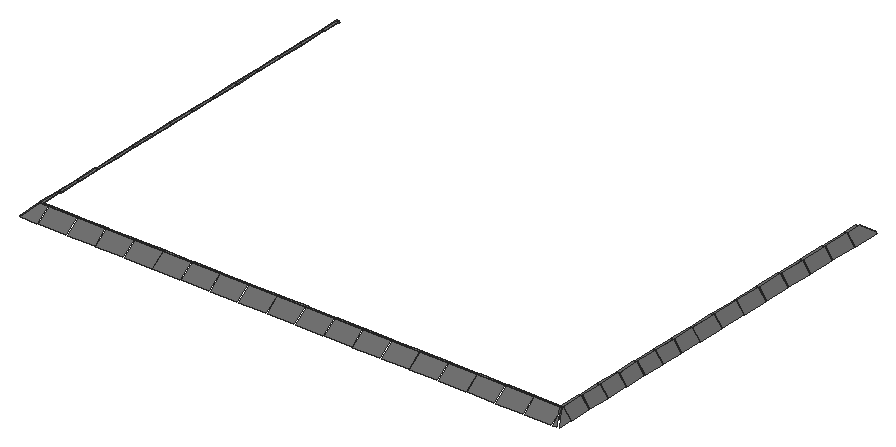
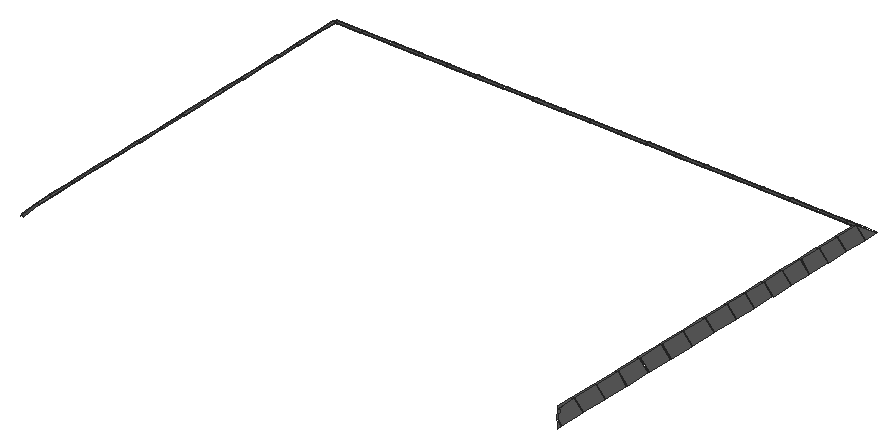
# SketchUp Ruby script. Lengths in inches.
U = 1.inch
M = Sketchup.active_model
def pt(a) = Geom::Point3d.new(a.map { |v| v * U })
def face(e, loops, mat)
  f = e.add_face(loops[0].map { |a| pt(a) })
  loops[1..].each { |l| e.add_face(l.map { |a| pt(a) }).erase! }
  f.material = f.back_material = mat if mat
  f
end
# faces: each face lists its corners as indices into pts; further lists are holes
def faces(e, pts, list, mat = nil) = list.each { |f| face(e, (f[0].is_a?(Array) ? f : [f]).map { |l| l.map { |i| pts[i] } }, mat) }
# xy, xz, yz: faces in a plane at the given z, y or x. An outline is a flat list of corners, or four numbers for a rectangle; further outlines are holes
def ring(l) = l.size == 4 ? [[l[0], l[1]], [l[2], l[1]], [l[2], l[3]], [l[0], l[3]]] : l.each_slice(2).to_a
def flat(e, list, mat, &to3) = list.each { |f| face(e, (f[0].is_a?(Array) ? f : [f]).map { |l| ring(l).map { |u, v| to3.(u, v) } }, mat) }
def xy(e, z, list, mat = nil) = flat(e, list, mat) { |x, y| [x, y, z] }
def xz(e, y, list, mat = nil) = flat(e, list, mat) { |x, z| [x, y, z] }
def yz(e, x, list, mat = nil) = flat(e, list, mat) { |y, z| [x, y, z] }
def lines(e, pts, list) = list.each { |a, b| e.add_line(pt(pts[a]), pt(pts[b])) }
# prism: a flat outline (further loops are holes) pulled along v
def prism(e, loops, v, mat = nil)
  f = face(e, loops, mat); d = Geom::Vector3d.new(v.map { |x| x * U })
  f.pushpull(f.normal.samedirection?(d) ? d.length : -d.length)
end
def box(e, o, s, mat = nil) = prism(e, [[o, [o[0] + s[0], o[1], o[2]], [o[0] + s[0], o[1] + s[1], o[2]], [o[0], o[1] + s[1], o[2]]]], [0, 0, s[2]], mat)
def at(x, y, z, deg = 0) = Geom::Transformation.translation(pt([x, y, z])) * Geom::Transformation.rotation(ORIGIN, Z_AXIS, deg.degrees)
def axes(o, x, y, z) = Geom::Transformation.new([*x, 0, *y, 0, *z, 0, *pt(o).to_a, 1])
def part(name) = M.definitions.add(name)
# library, detail: a bought-in or finely detailed component or shape, given as its bounding box
def library(name, o, s) = part(name).tap { |d| box(d.entities, o, s) }
def detail(e, o, s) = box(e.add_group.entities, o, s)
def put(e, d, t, mat = nil) = e.add_instance(d, t).tap { |i| i.material = mat if mat }
def group(e, t, mat = nil) = e.add_group.tap { |g| g.transformation = t; g.material = mat if mat }.entities
root = M.entities
M.materials.add("[Color M05]").color = [114, 114, 114]
p = [[790.34,286.64,408.32],[790.34,298,408.32],[783.88,298,416.64],[785.7,294.8,414.29],[787.2,292.16,412.36],[790.34,299.21,408.32],
  [790.34,317.375,408.32],[783.88,317.375,416.64],[783.88,299.21,416.64],[790.34,318.58,408.32],[790.34,336.74,408.32],[783.88,336.74,416.64],
  [783.88,318.58,416.64],[790.34,337.95,408.32],[790.34,356.11,408.32],[783.88,356.11,416.64],[783.88,337.95,416.64],[790.34,357.32,408.32],
  [790.34,375.48,408.32],[783.88,375.48,416.64],[783.88,357.32,416.64],[790.34,376.69,408.32],[790.34,394.85,408.32],[783.88,394.85,416.64],
  [783.88,376.69,416.64],[790.34,396.0625,408.32],[790.34,414.22,408.32],[783.88,414.22,416.64],[783.88,396.0625,416.64],[790.34,415.43,408.32],
  [790.34,433.59,408.32],[783.88,433.59,416.64],[783.88,415.43,416.64],[790.34,434.8,408.32],[790.34,456.8,408.32],[783.88,456.8,416.64],
  [783.88,434.8,416.64],[790.34,458.01,408.32],[790.34,480.02,408.32],[783.88,480.02,416.64],[783.88,458.01,416.64],[790.34,481.23,408.32],
  [790.34,503.23,408.32],[783.88,503.23,416.64],[783.88,481.23,416.64],[790.34,504.44,408.32],[790.34,526.45,408.32],[783.88,526.45,416.64],
  [783.88,504.44,416.64],[790.34,527.66,408.32],[790.34,549.66,408.32],[783.88,549.66,416.64],[783.88,527.66,416.64],[790.34,550.87,408.32],
  [790.34,572.875,408.32],[783.88,572.875,416.64],[783.88,550.87,416.64],[790.34,574.08,408.32],[790.34,596.09,408.32],[783.88,596.09,416.64],
  [783.88,574.08,416.64],[790.34,597.3,408.32],[790.34,619.3,408.32],[788.98,619.3,410.08],[783.88,610.34,416.64],[783.88,597.3,416.64],
  [336.88,286.64,408.43],[344.33,298,416.75],[336.88,298,408.43],[336.88,317.375,408.43],[336.88,299.21,408.43],[344.33,299.21,416.75],
  [344.33,317.375,416.75],[336.88,336.74,408.43],[336.88,318.58,408.43],[344.33,318.58,416.75],[344.33,336.74,416.75],[336.88,356.11,408.43],
  [336.88,337.95,408.43],[344.33,337.95,416.75],[344.33,356.11,416.75],[336.88,375.48,408.43],[336.88,357.32,408.43],[344.33,357.32,416.75],
  [344.33,375.48,416.75],[336.88,394.85,408.43],[336.88,376.69,408.43],[344.33,376.69,416.75],[344.33,394.85,416.75],[336.88,414.22,408.43],
  [336.88,396.0625,408.43],[344.33,396.0625,416.75],[344.33,414.22,416.75],[336.88,433.3,408.43],[336.88,415.43,408.43],[344.33,415.43,416.75],
  [344.33,433.3,416.75],[344.33,434.8,416.75],[344.33,456.21,416.75],[336.88,456.21,408.43],[336.88,434.8,408.43],[336.88,479.13,408.43],
  [336.88,457.71,408.43],[344.33,457.71,416.75],[344.33,479.13,416.75],[336.88,502.04,408.43],[336.88,480.63,408.43],[344.33,480.63,416.75],
  [344.33,502.04,416.75],[336.88,524.95,408.43],[336.88,503.54,408.43],[344.33,503.54,416.75],[344.33,524.95,416.75],[336.88,547.87,408.43],
  [336.88,526.45,408.43],[344.33,526.45,416.75],[344.33,547.87,416.75],[336.88,570.78,408.43],[336.88,549.37,408.43],[344.33,549.37,416.75],
  [344.33,570.78,416.75],[336.88,593.69,408.43],[336.88,572.28,408.43],[344.33,572.28,416.75],[344.33,593.69,416.75],[336.88,616.61,408.43],
  [336.88,595.19,408.43],[344.33,595.19,416.75],[344.33,610.34,416.75],[340.22,616.61,412.16],[336.88,621.71,408.43],[336.88,618.11,408.43],
  [339.24,618.11,411.06],[338.37,285.45,408.71],[352.12,285.45,408.71],[352.12,296.82,417.03],[345.82,296.82,417.03],[353.62,285.45,408.71],
  [376.12,285.45,408.71],[376.12,296.82,417.03],[353.62,296.82,417.03],[377.62,285.45,408.71],[400.12,285.45,408.71],[400.12,296.82,417.03],
  [377.62,296.82,417.03],[401.62,285.45,408.71],[424.12,285.45,408.71],[424.12,296.82,417.03],[401.62,296.82,417.03],[425.62,285.45,408.71],
  [448.12,285.45,408.71],[448.12,296.82,417.03],[425.62,296.82,417.03],[449.62,285.45,408.71],[472.12,285.45,408.71],[472.12,296.82,417.03],
  [449.62,296.82,417.03],[473.62,285.45,408.71],[496.12,285.45,408.71],[496.12,296.82,417.03],[473.62,296.82,417.03],[497.62,285.45,408.71],
  [520.12,285.45,408.71],[520.12,296.82,417.03],[497.62,296.82,417.03],[521.62,285.45,408.71],[544.12,285.45,408.71],[544.12,296.82,417.03],
  [521.62,296.82,417.03],[545.62,285.45,408.71],[568.12,285.45,408.71],[568.12,296.82,417.03],[545.62,296.82,417.03],[569.62,285.45,408.71],
  [592.12,285.45,408.71],[592.12,296.82,417.03],[569.62,296.82,417.03],[593.62,285.45,408.71],[616.15,285.45,408.71],[616.15,296.82,417.03],
  [593.62,296.82,417.03],[617.62,285.45,408.71],[640.12,285.45,408.71],[640.12,296.82,417.03],[617.62,296.82,417.03],[641.62,285.45,408.71],
  [664.12,285.45,408.71],[664.12,296.82,417.03],[641.62,296.82,417.03],[665.62,285.45,408.71],[688.12,285.45,408.71],[688.12,296.82,417.03],
  [665.62,296.82,417.03],[689.62,285.45,408.71],[712.12,285.45,408.71],[712.12,296.82,417.03],[689.62,296.82,417.03],[713.62,285.45,408.71],
  [736.12,285.45,408.71],[736.12,296.82,417.03],[713.62,296.82,417.03],[737.62,285.45,408.71],[760.12,285.45,408.71],[760.12,296.82,417.03],
  [737.62,296.82,417.03],[761.62,285.45,408.71],[784.12,285.45,408.71],[784.12,293.62,414.68],[782.3,296.82,417.03],[761.62,296.82,417.03],
  [788.76,285.45,408.71],[785.62,290.98,412.75],[785.62,285.45,408.71],[787.4,619.3,408.85],[782.3,610.34,415.41],[345.82,610.34,415.41],
  [341.71,616.61,410.82],[784.12,294.8,413.07],[785.62,292.16,411.14],[782.3,298,415.41],[352.12,298,415.41],[345.82,298,415.41],
  [376.12,298,415.41],[353.62,298,415.41],[400.12,298,415.41],[377.62,298,415.41],[424.12,298,415.41],[401.62,298,415.41],
  [448.12,298,415.41],[425.62,298,415.41],[472.12,298,415.41],[449.62,298,415.41],[496.12,298,415.41],[473.62,298,415.41],
  [520.12,298,415.41],[497.62,298,415.41],[544.12,298,415.41],[521.62,298,415.41],[568.12,298,415.41],[545.62,298,415.41],
  [592.12,298,415.41],[569.62,298,415.41],[616.15,298,415.41],[593.62,298,415.41],[640.12,298,415.41],[617.62,298,415.41],
  [664.12,298,415.41],[641.62,298,415.41],[688.12,298,415.41],[665.62,298,415.41],[712.12,298,415.41],[689.62,298,415.41],
  [736.12,298,415.41],[713.62,298,415.41],[760.12,298,415.41],[737.62,298,415.41],[761.62,298,415.41],[352.12,299.21,416.3],
  [346.61,299.21,416.3],[345.82,299.21,415.41],[353.62,299.21,416.3],[376.12,299.21,416.3],[377.62,299.21,416.3],[400.12,299.21,416.3],
  [401.62,299.21,416.3],[424.12,299.21,416.3],[425.62,299.21,416.3],[448.12,299.21,416.3],[449.62,299.21,416.3],[472.12,299.21,416.3],
  [473.62,299.21,416.3],[496.12,299.21,416.3],[497.62,299.21,416.3],[520.12,299.21,416.3],[521.62,299.21,416.3],[544.12,299.21,416.3],
  [545.62,299.21,416.3],[568.12,299.21,416.3],[569.62,299.21,416.3],[592.12,299.21,416.3],[593.62,299.21,416.3],[616.15,299.21,416.3],
  [617.62,299.21,416.3],[640.12,299.21,416.3],[641.62,299.21,416.3],[664.12,299.21,416.3],[665.62,299.21,416.3],[688.12,299.21,416.3],
  [689.62,299.21,416.3],[712.12,299.21,416.3],[713.62,299.21,416.3],[736.12,299.21,416.3],[737.62,299.21,416.3],[760.12,299.21,416.3],
  [761.62,299.21,416.3],[781.61,299.21,416.3],[782.3,299.21,415.41],[345.82,317.375,415.41],[346.61,317.375,416.3],[782.3,317.375,415.41],
  [781.61,317.375,416.3],[345.82,318.58,415.41],[346.61,318.58,416.3],[782.3,318.58,415.41],[781.61,318.58,416.3],[345.82,336.74,415.41],
  [346.61,336.74,416.3],[782.3,336.74,415.41],[781.61,336.74,416.3],[345.82,337.95,415.41],[346.61,337.95,416.3],[782.3,337.95,415.41],
  [781.61,337.95,416.3],[345.82,356.11,415.41],[346.61,356.11,416.3],[782.3,356.11,415.41],[781.61,356.11,416.3],[345.82,357.32,415.41],
  [346.61,357.32,416.3],[782.3,357.32,415.41],[781.61,357.32,416.3],[345.82,375.48,415.41],[346.61,375.48,416.3],[782.3,375.48,415.41],
  [781.61,375.48,416.3],[346.61,376.69,416.3],[345.82,376.69,415.41],[782.3,376.69,415.41],[781.61,376.69,416.3],[345.82,394.85,415.41],
  [346.61,394.85,416.3],[782.3,394.85,415.41],[781.61,394.85,416.3],[345.82,396.0625,415.41],[346.61,396.0625,416.3],[782.3,396.0625,415.41],
  [781.61,396.0625,416.3],[345.82,414.22,415.41],[346.61,414.22,416.3],[782.3,414.22,415.41],[781.61,414.22,416.3],[345.82,415.43,415.41],
  [346.61,415.43,416.3],[782.3,415.43,415.41],[781.61,415.43,416.3],[345.82,433.3,415.41],[346.61,433.3,416.3],[782.3,433.59,415.41],
  [781.61,433.59,416.3],[345.82,434.8,415.41],[346.61,434.8,416.3],[782.3,434.8,415.41],[781.61,434.8,416.3],[345.82,456.21,415.41],
  [346.61,456.21,416.3],[782.3,456.8,415.41],[781.61,456.8,416.3],[345.82,457.71,415.41],[346.61,457.71,416.3],[782.3,458.01,415.41],
  [781.61,458.01,416.3],[345.82,479.13,415.41],[346.61,479.13,416.3],[782.3,480.02,415.41],[781.61,480.02,416.3],[345.82,480.63,415.41],
  [346.61,480.63,416.3],[782.3,481.23,415.41],[781.61,481.23,416.3],[345.82,502.04,415.41],[346.61,502.04,416.3],[782.3,503.23,415.41],
  [781.61,503.23,416.3],[345.82,503.54,415.41],[346.61,503.54,416.3],[782.3,504.44,415.41],[781.61,504.44,416.3],[345.82,524.95,415.41],
  [346.61,524.95,416.3],[782.3,526.45,415.41],[781.61,526.45,416.3],[345.82,526.45,415.41],[346.61,526.45,416.3],[782.3,527.66,415.41],
  [781.61,527.66,416.3],[345.82,547.87,415.41],[346.61,547.87,416.3],[782.3,549.66,415.41],[781.61,549.66,416.3],[345.82,549.37,415.41],
  [346.61,549.37,416.3],[345.82,570.78,415.41],[346.61,570.78,416.3],[782.3,550.87,415.41],[781.61,550.87,416.3],[782.3,572.875,415.41],
  [781.61,572.875,416.3],[345.82,572.28,415.41],[346.61,572.28,416.3],[345.82,593.69,415.41],[346.61,593.69,416.3],[782.3,574.08,415.41],
  [781.61,574.08,416.3],[782.3,596.09,415.41],[781.61,596.09,416.3],[345.82,595.19,415.41],[346.61,595.19,416.3],[346.61,609.125,416.3],
  [782.3,597.3,415.41],[781.61,597.3,416.3],[781.61,609.125,416.3]]
faces(root,p,[[0,1,2,3,4],[5,6,7,8],[9,10,11,12],[13,14,15,16],[17,18,19,20],[21,22,23,24],[25,26,27,28],[29,30,31,32],
  [33,34,35,36],[37,38,39,40],[41,42,43,44],[45,46,47,48],[49,50,51,52],[53,54,55,56],[57,58,59,60],[61,62,63,64,65],
  [66,67,68],[69,70,71,72],[73,74,75,76],[77,78,79,80],[81,82,83,84],[85,86,87,88],[89,90,91,92],[93,94,95,96],
  [97,98,99,100],[101,102,103,104],[105,106,107,108],[109,110,111,112],[113,114,115,116],[117,118,119,120],[121,122,123,124],[125,126,127,128,129],
  [130,131,132],[133,134,135,136],[137,138,139,140],[141,142,143,144],[145,146,147,148],[149,150,151,152],[153,154,155,156],[157,158,159,160],
  [161,162,163,164],[165,166,167,168],[169,170,171,172],[173,174,175,176],[177,178,179,180],[181,182,183,184],[185,186,187,188],[189,190,191,192],
  [193,194,195,196],[197,198,199,200],[201,202,203,204],[205,206,207,208,209],[210,211,212],[213,214,64,63],[215,216,129,128],[217,218,4,3],
  [217,219,208,207],[219,217,3,2],[220,221,136,135],[222,223,140,139],[224,225,144,143],[226,227,148,147],[228,229,152,151],[230,231,156,155],
  [232,233,160,159],[234,235,164,163],[236,237,168,167],[238,239,172,171],[240,241,176,175],[242,243,180,179],[244,245,184,183],[246,247,188,187],
  [248,249,192,191],[250,251,196,195],[252,253,200,199],[254,255,204,203],[219,256,209,208],[221,220,257,258],[221,258,259],[220,223,260,257],
  [223,222,261,260],[222,225,262,261],[225,224,263,262],[224,227,264,263],[227,226,265,264],[226,229,266,265],[229,228,267,266],[228,231,268,267],
  [231,230,269,268],[230,233,270,269],[233,232,271,270],[232,235,272,271],[235,234,273,272],[234,237,274,273],[237,236,275,274],[236,239,276,275],
  [239,238,277,276],[238,241,278,277],[241,240,279,278],[240,243,280,279],[243,242,281,280],[242,245,282,281],[245,244,283,282],[244,247,284,283],
  [247,246,285,284],[246,249,286,285],[249,248,287,286],[248,251,288,287],[251,250,289,288],[250,253,290,289],[253,252,291,290],[252,255,292,291],
  [255,254,293,292],[254,256,294,293],[295,294,256,219],[295,219,296],[259,297,72,71],[297,259,258,298],[296,299,300,295],[299,296,8,7],
  [301,297,298,302],[299,303,304,300],[301,305,76,75],[305,301,302,306],[303,307,308,304],[307,303,12,11],[309,305,306,310],[307,311,312,308],
  [309,313,80,79],[313,309,310,314],[311,315,316,312],[315,311,16,15],[317,313,314,318],[315,319,320,316],[317,321,84,83],[321,317,318,322],
  [319,323,324,320],[323,319,20,19],[322,325,326,321],[323,327,328,324],[326,329,88,87],[329,326,325,330],[327,331,332,328],[331,327,24,23],
  [333,329,330,334],[331,335,336,332],[333,337,92,91],[337,333,334,338],[335,339,340,336],[339,335,28,27],[341,337,338,342],[339,343,344,340],
  [341,345,96,95],[345,341,342,346],[343,347,348,344],[347,343,32,31],[349,345,346,350],[347,351,352,348],[349,353,98,97],[350,354,353,349],
  [351,355,356,352],[355,351,36,35],[357,353,354,358],[355,359,360,356],[357,361,104,103],[361,357,358,362],[359,363,364,360],[363,359,40,39],
  [365,361,362,366],[363,367,368,364],[365,369,108,107],[369,365,366,370],[367,371,372,368],[371,367,44,43],[373,369,370,374],[371,375,376,372],
  [373,377,112,111],[377,373,374,378],[375,379,380,376],[379,375,48,47],[381,377,378,382],[379,383,384,380],[381,385,116,115],[385,381,382,386],
  [383,387,388,384],[387,383,52,51],[389,385,386,390],[389,391,120,119],[391,389,390,392],[387,393,394,388],[393,395,396,394],[395,393,56,55],
  [397,391,392,398],[397,399,124,123],[399,397,398,400],[395,401,402,396],[401,403,404,402],[403,401,60,59],[405,399,400,406],[405,215,128,127],
  [215,405,406,407],[403,408,409,404],[410,409,408,214],[214,408,65,64]],"[Color M05]")
